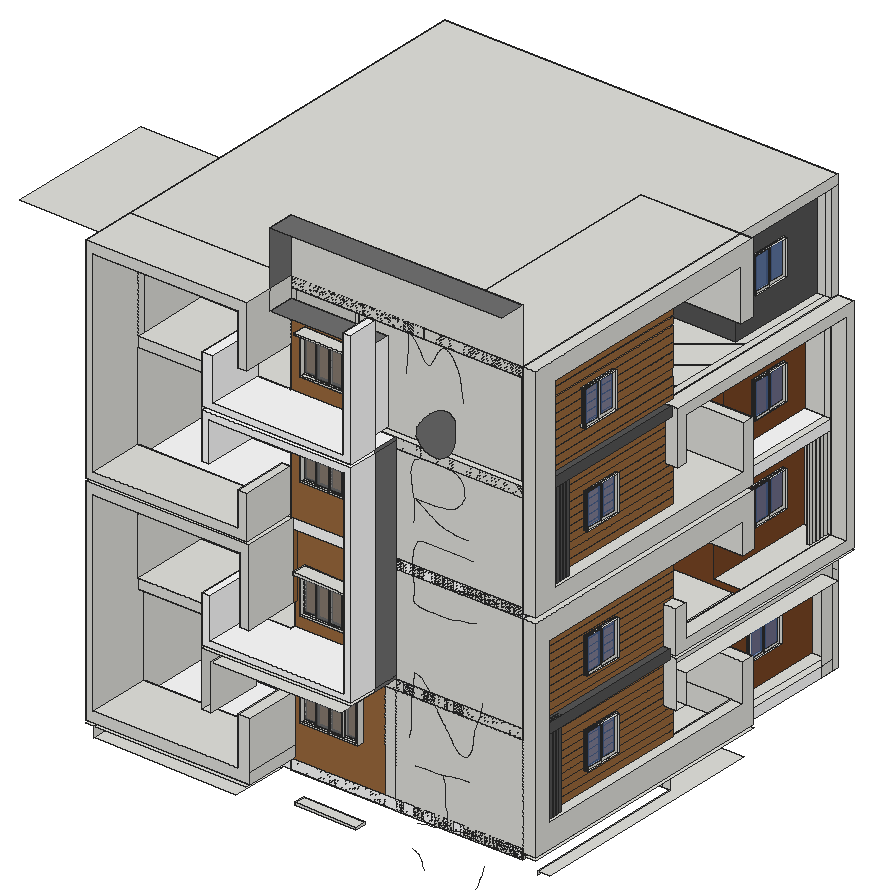
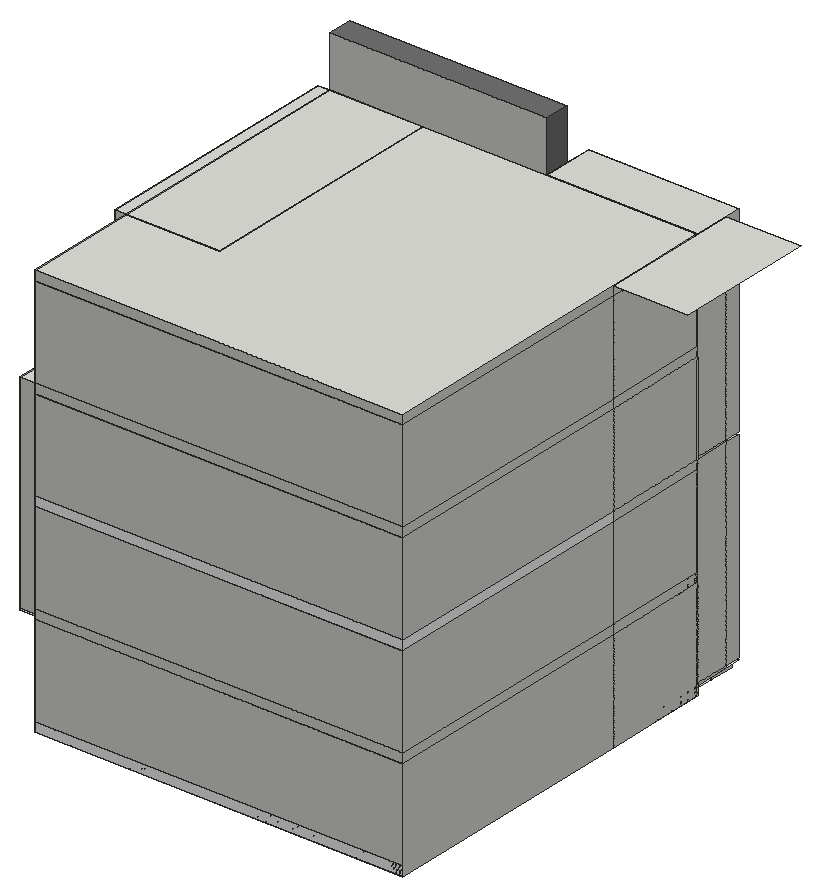
# SketchUp Ruby script. Lengths in inches.
U = 1.inch
M = Sketchup.active_model
def pt(a) = Geom::Point3d.new(a.map { |v| v * U })
def face(e, loops, mat)
  f = e.add_face(loops[0].map { |a| pt(a) })
  loops[1..].each { |l| e.add_face(l.map { |a| pt(a) }).erase! }
  f.material = f.back_material = mat if mat
  f
end
# faces: each face lists its corners as indices into pts; further lists are holes
def faces(e, pts, list, mat = nil) = list.each { |f| face(e, (f[0].is_a?(Array) ? f : [f]).map { |l| l.map { |i| pts[i] } }, mat) }
# xy, xz, yz: faces in a plane at the given z, y or x. An outline is a flat list of corners, or four numbers for a rectangle; further outlines are holes
def ring(l) = l.size == 4 ? [[l[0], l[1]], [l[2], l[1]], [l[2], l[3]], [l[0], l[3]]] : l.each_slice(2).to_a
def flat(e, list, mat, &to3) = list.each { |f| face(e, (f[0].is_a?(Array) ? f : [f]).map { |l| ring(l).map { |u, v| to3.(u, v) } }, mat) }
def xy(e, z, list, mat = nil) = flat(e, list, mat) { |x, y| [x, y, z] }
def xz(e, y, list, mat = nil) = flat(e, list, mat) { |x, z| [x, y, z] }
def yz(e, x, list, mat = nil) = flat(e, list, mat) { |y, z| [x, y, z] }
def lines(e, pts, list) = list.each { |a, b| e.add_line(pt(pts[a]), pt(pts[b])) }
# prism: a flat outline (further loops are holes) pulled along v
def prism(e, loops, v, mat = nil)
  f = face(e, loops, mat); d = Geom::Vector3d.new(v.map { |x| x * U })
  f.pushpull(f.normal.samedirection?(d) ? d.length : -d.length)
end
def box(e, o, s, mat = nil) = prism(e, [[o, [o[0] + s[0], o[1], o[2]], [o[0] + s[0], o[1] + s[1], o[2]], [o[0], o[1] + s[1], o[2]]]], [0, 0, s[2]], mat)
def at(x, y, z, deg = 0) = Geom::Transformation.translation(pt([x, y, z])) * Geom::Transformation.rotation(ORIGIN, Z_AXIS, deg.degrees)
def axes(o, x, y, z) = Geom::Transformation.new([*x, 0, *y, 0, *z, 0, *pt(o).to_a, 1])
def part(name) = M.definitions.add(name)
# library, detail: a bought-in or finely detailed component or shape, given as its bounding box
def library(name, o, s) = part(name).tap { |d| box(d.entities, o, s) }
def detail(e, o, s) = box(e.add_group.entities, o, s)
def put(e, d, t, mat = nil) = e.add_instance(d, t).tap { |i| i.material = mat if mat }
def group(e, t, mat = nil) = e.add_group.tap { |g| g.transformation = t; g.material = mat if mat }.entities
root = M.entities
M.materials.add("[Color M00]").color = [255, 255, 255]
M.materials.add("[Color M05]").color = [114, 114, 114]
M.materials.add("[Color M06]").color = [86, 86, 86]
M.materials.add("[Translucent Glass Blue]").color = [100, 149, 237]
M.materials["[Translucent Glass Blue]"].alpha = 0.5
M.materials.add("[Translucent_Glass_Gray]").color = [128, 128, 128]
M.materials["[Translucent_Glass_Gray]"].alpha = 0.5
M.materials.add("[Wood Floor]").color = [155, 105, 61]
M.materials.add("[Wood Veneer 01]").color = [120, 70, 37]
M.materials.add("[Wood Veneer 02]").color = [190, 128, 91]
c1 = part("Group\#4")
box(c1.entities,[0,-480,0],[480,480,12])
c2 = part("Janela aluminio")
xy(c2.entities,0,[[0,0,47.24,1.57],[23.62,1.57,47.24,2.76],[0,2.76,25.98,3.9375],[0,3.9375,47.24,5.91]])
xy(c2.entities,43.31,[[0,0,47.24,1.57],[23.62,1.57,47.24,2.76],[0,2.76,0,5.91,47.24,5.91,47.24,3.9375,25.98,3.9375,25.98,2.76],[25.98,2.76,47.24,3.9375]])
xz(c2.entities,1.57,[[0,0,23.62,0,23.62,41.34,21.26,41.34,21.26,1.97,1.97,1.97,1.97,41.34,23.62,41.34,23.62,43.31,0,43.31],[[23.62,0,47.24,43.31],[25.7,1.97,45.28,41.34]]])
xz(c2.entities,2.76,[[[0,0,23.62,43.31],[2.36,2.36,21.26,40.94]],[23.62,0,25.98,43.31]])
xz(c2.entities,2.76,[[2.36,2.36,21.26,40.94]],"[Translucent Glass Blue]")
xz(c2.entities,3.9375,[[25.98,0,25.98,2.36,44.88,2.36,44.88,40.94,25.98,40.94,25.98,43.31,47.24,43.31,47.24,0]])
xz(c2.entities,3.9375,[[25.98,2.36,44.88,40.94]],"[Translucent Glass Blue]")
yz(c2.entities,0,[[0,0,1.57,43.31],[2.76,0,5.91,43.31]])
yz(c2.entities,23.62,[[1.57,0,2.76,43.31]])
yz(c2.entities,25.98,[[2.76,0,3.9375,43.31]])
yz(c2.entities,47.24,[[0,0,1.57,43.31],[1.57,0,2.76,43.31],[3.9375,0,5.91,43.31]])
c3 = part("Group\#11")
box(c3.entities,[0,0,0],[3.1875,2.5625,106.5625],"[Color M06]")
c4 = part("Group\#5")
xy(c4.entities,0,[[0,0,3.25,201.7]])
xy(c4.entities,8.11,[[0,0,3.25,201.7]])
xz(c4.entities,201.7,[[0,0,3.25,8.11]])
yz(c4.entities,3.25,[[0,0,201.7,8.11]])
c5 = part("Window frame")
prism(c5.entities,[[[0,70.87,0],[0,0,0],[0,0,47.24],[0,70.87,47.24]],[[0,1.97,1.97],[0,68.9,1.97],[0,68.9,45.28],[0,1.97,45.28]]],[7.875,0,0])
c6 = part("Window sash")
xy(c6.entities,0,[[0,0,3.9375,16.73]])
xy(c6.entities,0.98,[[0,0.98,1.77,15.75],[1.77,0.98,2.85,15.75],[2.85,0.98,3.9375,15.75]])
xy(c6.entities,42.32,[[0,0.98,1.77,15.75],[1.77,0.98,2.85,15.75],[2.85,0.98,3.9375,15.75]])
xy(c6.entities,43.31,[[0,0,3.9375,16.73]])
xz(c6.entities,0,[[0,0,3.9375,43.31]])
xz(c6.entities,0.98,[[0,0.98,1.77,42.32],[1.77,0.98,2.85,42.32],[2.85,0.98,3.9375,42.32]])
xz(c6.entities,15.75,[[0,0.98,1.77,42.32],[1.77,0.98,2.85,42.32],[2.85,0.98,3.9375,42.32]])
xz(c6.entities,16.73,[[0,0,3.9375,43.31]])
yz(c6.entities,0,[[[0,0,16.73,43.31],[0.98,0.98,15.75,42.32]]])
yz(c6.entities,1.77,[[0.98,0.98,15.75,42.32]],"[Translucent_Glass_Gray]")
yz(c6.entities,2.85,[[0.98,0.98,15.75,42.32]],"[Translucent_Glass_Gray]")
yz(c6.entities,3.9375,[[[0,0,16.73,43.31],[0.98,0.98,15.75,42.32]]])
c7 = part("simple window")
p = [[0,68.9,1.97],[0,35.43,1.97]]
lines(c7.entities,p,[[0,1]])
put(c7.entities,c5,at(0,0,0))
put(c7.entities,c6,axes([1.14,52.17,1.97],[0.71,0,0],[0,1,0],[0,0,1]))
put(c7.entities,c6,axes([1.14,1.97,1.97],[0.71,0,0],[0,1,0],[0,0,1]))
put(c7.entities,c6,axes([3.9375,18.7,1.97],[0.71,0,0],[0,1,0],[0,0,1]))
put(c7.entities,c6,axes([3.9375,35.43,1.97],[0.71,0,0],[0,1,0],[0,0,1]))
c8 = part("Group\#12")
box(c8.entities,[0,0,-113.625],[4.125,3.0625,113.625])
prism(root,[[[309.42,176.67,224.48],[385.14,174.47,224.48],[384.74,160.72,224.48],[309.02,162.93,224.48]]],[0,0,2.95])
prism(root,[[[310.01,176.625,477.8],[385.52,174.46,477.8],[385.01,156.71,477.8],[309.5,158.88,477.8]]],[0,0,3.17])
prism(root,[[[309.78,176.625,739.55],[382.52,174.54,739.55],[382.09,159.42,739.55],[309.34,161.5,739.55]]],[0,0,2.58])
xy(root,230.57,[[576.8125,198.69,576.8125,400.39,441.125,400.39,441.125,495.37,591.75,495.37,591.75,198.69]])
xy(root,251.42,[[282.85,105.86,106.76,108.5,107.25,141,107.25,141.5625,107.78,176.625,283.87,173.99],[106.75,108.5,107.25,141.5625,107.25,141,106.76,108.5]])
xy(root,252,[[96.8125,176.625,96.8125,656.625,576.8125,656.625,576.8125,647.625,441.125,647.625,441.125,400.39,576.8125,400.39,576.8125,176.625,293.58,176.625,293.58,273.5625,105.8125,273.5625,105.8125,176.625],[441.125,400.39,576.8125,509.52],[441.125,509.52,552.625,647.625]])
xy(root,256.375,[[576.8125,176.625,591.75,509.52]])
xy(root,260.25,[[576.8125,176.625,591.75,508.3125]])
xy(root,264,[[294.92,105.68,295.94,173.81,107.78,176.625,107.25,176.625,107.25,108.5,106.76,108.5],[96.8125,108.5,106.75,108.5,107.25,141.5625,107.25,176.625,96.8125,176.625],[106.75,108.5,106.76,108.5,107.25,141,107.25,141.5625],[106.76,108.5,107.25,108.5,107.25,141],[105.8125,176.625,107.25,176.75],
  [368.4,185.625,567.8125,185.625,567.8125,391.39,432.125,391.39,432.125,647.625,105.8125,647.625,105.8125,282.5625,368.4,282.5625],[441.125,400.39,567.8125,493.4],[567.8125,400.39,576.8125,493.4],[441.125,493.4,567.8125,508.3125],[567.8125,493.4,576.8125,508.3125],
  [441.125,508.3125,552.625,647.625],[552.625,508.3125,567.8125,647.625],[567.8125,508.3125,576.8125,647.625]])
xy(root,266.9,[[96.8125,108.5,297.75,176.625],[105.8125,176.625,297.75,185.625]])
xy(root,280.02,[[105.8125,108.5,282.85,185.625]])
xy(root,289.03,[[576.8125,196.5,591.75,493.4]])
xy(root,328.5625,[[238.96,108.5,250.4375,176.625]])
xy(root,331.1,[[576.8125,385.5625,596.375,400.39]])
xy(root,335.41,[[441.125,493.4,591.75,508.3125]])
xy(root,338.39,[[282.85,108.5,297.75,185.625]])
xy(root,365.16,[[576.8125,400.39,596.375,631.75]])
xy(root,384,[[250.4375,108.5,408.47,176.625],[[96.8125,176.625,105.8125,176.625,105.8125,273.5625,293.58,273.5625,293.58,176.625,576.8125,176.625,576.8125,400.39,441.125,400.39,441.125,508.3125,552.625,508.3125,552.625,647.625,576.8125,647.625,576.8125,656.625,96.8125,656.625],[368.4,185.625,368.4,282.5625,105.8125,282.5625,105.8125,647.625,432.125,647.625,432.125,391.39,567.8125,391.39,567.8125,185.625]]])
xy(root,384,[[576.8125,196.5,589.1875,385.5625]],"[Color M06]")
xy(root,387.92,[[576.8125,385.5625,596.375,656.625]])
xy(root,390.25,[[576.8125,385.5625,596.375,656.7]])
xy(root,396,[[238.96,108.5,421.4,176.625],[[96.8125,176.625,105.8125,176.625,105.8125,273.5625,293.58,273.5625,293.58,176.625,576.8125,176.625,576.8125,400.39,441.125,400.39,441.125,508.3125,576.8125,508.3125,576.8125,656.625,96.8125,656.625],[368.4,185.625,368.4,282.5625,105.8125,282.5625,105.8125,647.625,432.125,647.625,432.125,391.39,567.8125,391.39,567.8125,185.625]],[105.8125,176.625,293.58,273.5625],[368.4,185.625,567.8125,185.625,567.8125,391.39,432.125,391.39,432.125,647.625,105.8125,647.625,105.8125,282.5625,368.4,282.5625],[441.125,400.39,567.8125,508.3125],
  [567.8125,400.39,576.8125,508.3125]])
xy(root,396,[[576.8125,196.5,589.1875,385.5625]],"[Color M06]")
xy(root,399.23,[[238.96,108.5,421.4,176.625]],"[Color M00]")
xy(root,402.375,[[576.8125,400.39,596.375,645.5],[543.8125,508.3125,576.8125,645.5]])
xy(root,406.73,[[248.78,108.5,412.35,108.5,412.35,181.6875,293.58,181.6875,293.58,176.625,248.78,176.625]],"[Color M00]")
xy(root,434.5625,[[284.9,108.5,295.8125,176.625]])
xy(root,434.5625,[[293.58,176.625,295.8125,181.6875]],"[Wood Floor]")
xy(root,442.24,[[576.8125,385.5625,596.375,400.39]])
xy(root,451.24,[[443.1875,493.73,591.75,509.52]])
xy(root,455.73,[[238.96,108.5,248.78,176.625]],"[Color M00]")
xy(root,488.49,[[576.8125,196.5,576.8125,400.39,443.1875,400.39,443.1875,493.73,591.75,493.73,591.75,196.5]])
xy(root,516,[[105.8125,108.5,284.9,176.625],[[96.8125,176.625,105.8125,176.625,105.8125,273.5625,293.58,273.5625,293.58,176.625,295.8125,176.625,295.8125,181.6875,412.35,181.6875,412.35,176.625,576.8125,176.625,576.8125,400.39,441.125,400.39,441.125,508.3125,543.8125,508.3125,543.8125,645.5,576.8125,645.5,576.8125,656.625,96.8125,656.625],[368.4,185.625,368.4,282.5625,105.8125,282.5625,105.8125,647.625,432.125,647.625,432.125,391.39,567.8125,391.39,567.8125,185.625]],[105.8125,176.625,293.58,273.5625]])
xy(root,516.375,[[576.8125,176.625,591.75,176.625,591.75,509.52,443.1875,509.52,443.1875,400.39,576.8125,400.39]])
xy(root,522,[[576.8125,176.625,591.75,508.3125]])
xy(root,528,[[96.8125,108.5,295.8125,176.625],[[96.8125,176.625,105.8125,176.625,105.8125,273.5625,293.58,273.5625,293.58,176.625,576.8125,176.625,576.8125,400.39,441.125,400.39,441.125,524.01,543.8125,524.01,543.8125,647.625,576.8125,647.625,576.8125,656.625,96.8125,656.625],[368.4,185.625,368.4,282.5625,105.8125,282.5625,105.8125,647.625,432.125,647.625,432.125,391.39,567.8125,391.39,567.8125,185.625]],[368.4,185.625,567.8125,185.625,567.8125,391.39,432.125,391.39,432.125,647.625,105.8125,647.625,105.8125,282.5625,368.4,282.5625],[441.125,400.39,452.75,400.39,452.75,508.3125,567.8125,508.3125,567.8125,647.625,543.8125,647.625,543.8125,524.01,441.125,524.01],[452.75,400.39,567.8125,508.3125],
  [567.8125,400.39,576.8125,508.3125],[567.8125,508.3125,576.8125,647.625]])
xy(root,531.25,[[96.8125,108.5,293.58,176.625]])
xy(root,541.94,[[105.8125,108.5,282.6,176.625]])
xy(root,542.625,[[576.8125,206.2,591.75,206.2,591.75,494.4,452.75,494.4,452.75,400.39,576.8125,400.39]])
xy(root,583.51,[[282.6,108.5,293.58,176.625]])
xy(root,595.125,[[576.8125,388.1875,596.375,400.39]])
xy(root,596.1875,[[452.75,494.4,591.75,508.3125]])
xy(root,599.8125,[[238.96,108.5,247.93,176.625]],"[Color M00]")
xy(root,648,[[[96.8125,176.625,105.8125,176.625,105.8125,273.5625,293.58,273.5625,293.58,176.625,576.8125,176.625,576.8125,400.39,441.125,400.39,441.125,524.01,543.8125,524.01,543.8125,647.625,576.8125,647.625,576.8125,656.625,96.8125,656.625],[368.4,185.625,368.4,282.5625,105.8125,282.5625,105.8125,647.625,432.125,647.625,432.125,391.39,567.8125,391.39,567.8125,185.625]],[576.8125,400.39,596.375,645.5]])
xy(root,648,[[247.93,108.5,412.35,176.625]],"[Color M00]")
xy(root,648,[[576.8125,206.2,588.625,388.1875]],"[Color M06]")
xy(root,656.3125,[[238.96,108.5,421.4,176.625]],"[Color M00]")
xy(root,660,[[[96.8125,176.625,105.8125,176.625,105.8125,273.5625,293.58,273.5625,293.58,176.625,576.8125,176.625,576.8125,400.39,441.125,400.39,441.125,524.01,558.6875,524.01,558.6875,647.625,576.8125,647.625,576.8125,656.625,96.8125,656.625],[368.4,185.625,368.4,282.5625,105.8125,282.5625,105.8125,647.625,432.125,647.625,432.125,391.39,567.8125,391.39,567.8125,185.625]],[105.8125,176.625,293.58,273.5625],[368.4,185.625,567.8125,185.625,567.8125,391.39,432.125,391.39,432.125,647.625,105.8125,647.625,105.8125,282.5625,368.4,282.5625],[576.8125,388.1875,596.375,656.7],[441.125,400.39,567.8125,400.39,567.8125,647.625,558.6875,647.625,558.6875,524.01,441.125,524.01],
  [567.8125,400.39,576.8125,647.625]])
xy(root,660,[[576.8125,206.2,588.625,388.1875]],"[Color M06]")
xy(root,660.31,[[238.96,108.5,421.4,176.625]],"[Color M00]")
xy(root,667.83,[[252.22,108.5,411.47,176.625]],"[Color M00]")
xy(root,706.5625,[[455.0625,490.39,591.75,508.3125]])
xy(root,717.3125,[[283.44,108.5,293.58,176.625]])
xy(root,719.51,[[238.96,108.5,252.22,176.625]],"[Color M00]")
xy(root,767.74,[[293.58,144.25,411.47,176.625]],"[Color M05]")
xy(root,768.8125,[[576.8125,206.2,576.8125,400.39,455.0625,400.39,455.0625,490.39,591.75,490.39,591.75,206.2]])
xy(root,780,[[105.8125,108.5,283.44,176.625],[96.8125,176.625,105.8125,176.625,105.8125,273.5625,293.58,273.5625,293.58,176.625,455.0625,176.625,455.0625,185.625,368.4,185.625,368.4,282.5625,105.8125,282.5625,105.8125,647.625,432.125,647.625,432.125,391.39,455.0625,391.39,455.0625,400.39,441.125,400.39,441.125,524.01,558.6875,524.01,558.6875,647.625,576.8125,647.625,576.8125,656.625,96.8125,656.625],[455.0625,176.625,576.8125,176.625,576.8125,400.39,455.0625,400.39,455.0625,391.39,567.8125,391.39,567.8125,185.625,455.0625,185.625],[455.0625,185.625,567.8125,391.39]])
xy(root,792,[[96.8125,108.5,293.58,176.625],[0,129.5,96.8125,313.4],[455.0625,176.625,591.75,508.3125]])
xy(root,801.24,[[411.47,108.5,421.4,144.25]],"[Color M00]")
xy(root,859.0625,[[293.58,144.25,576.8125,176.625]],"[Color M05]")
xz(root,108.5,[[96.8125,266.9,297.75,266.9,297.75,338.39,282.85,338.39,282.85,280.02,105.8125,280.02,105.8125,516,284.9,516,284.9,434.5625,295.8125,434.5625,295.8125,528,96.8125,528],[96.8125,531.25,293.58,531.25,293.58,583.51,282.6,583.51,282.6,541.94,105.8125,541.94,105.8125,780,283.44,780,283.44,717.3125,293.58,717.3125,293.58,792,96.8125,792]])
xz(root,108.5,[[238.96,399.23,421.4,399.23,421.4,656.3125,238.96,656.3125,238.96,599.8125,247.93,599.8125,247.93,648,412.35,648,412.35,406.73,248.78,406.73,248.78,455.73,238.96,455.73],[238.96,660.31,421.4,660.31,421.4,801.24,411.47,801.24,411.47,667.83,252.22,667.83,252.22,719.51,238.96,719.51]],"[Color M00]")
xz(root,144.25,[[499.28,678.61,502.39,679.59,504.6,680.79,507.3125,682.48,509.4,683.71,511.65,685.61,512.91,687.64,514.6,689.38,515.95,691.83,517.19,693.71,518.06,696.2,518.48,698.83,518.75,701.49,518.93,703.9,519.01,706.6,519.06,709.68,519.08,712.16,519.08,715.27,519.07,717.8,519.05,720.89,519.03,723.43,518.67,726.53,517.58,728.38,515.96,730.33,513.8,731.55,511.41,732.18,508.87,732.625,506.22,732.9,498.73,730.52,494.25,727.71,489.21,724.33,488.32,722.59,486.18,720.94,484.83,719.08,482.91,717.36,481.51,715.31,479.9,713.53,478.57,711.1,477,709.55,475.72,707.47,474.84,705.29,473.375,703.48,472.87,700.99,472.54,698.74,472.29,696.5,472.16,693.875,473.78,691.2,475.09,689.5,476.52,686.92,478.12,684.95,480.42,683.44,481.86,681.66,483.9,680.62,486.04,679.74,488.85,679.28,491.18,678.99,493.5,678.8,496.52,678.68]],"[Color M05]")
xz(root,176.625,[[96.8125,252,105.8125,264],[408.47,252,421.4,384],[421.4,252,576.8125,384],[576.8125,260.25,591.75,516.375],[96.8125,264,105.8125,266.9],
  [238.96,328.5625,238.96,396,421.4,396,421.4,384,250.4375,384,250.4375,328.5625],[96.8125,384,105.8125,396],[421.4,384,576.8125,396],[421.4,396,576.8125,516],[284.9,434.5625,293.58,516],
  [293.58,434.5625,295.8125,516],[96.8125,516,295.8125,528],[421.4,516,576.8125,528],[576.8125,522,591.75,792],[96.8125,528,105.8125,531.25],
  [421.4,528,576.8125,648],[105.8125,531.25,105.8125,541.94,282.6,541.94,282.6,583.51,293.58,583.51,293.58,531.25],[96.8125,648,105.8125,660],[421.4,648,576.8125,660],[96.8125,660,105.8125,780],
  [283.44,717.3125,283.44,780,96.8125,780,96.8125,792,293.58,792,293.58,717.3125],[293.58,780,293.58,859.0625,576.8125,859.0625,576.8125,792,455.0625,792,455.0625,780],[455.0625,780,576.8125,792]])
xz(root,176.625,[[412.35,516,421.4,528],[238.96,599.8125,238.96,656.3125,421.4,656.3125,421.4,648,247.93,648,247.93,599.8125]],"[Color M00]")
xz(root,176.625,[[293.58,252,408.47,384],[293.58,396,421.4,399.23],[238.96,399.23,238.96,455.73,248.78,455.73,248.78,406.73,293.58,406.73,293.58,399.23],[293.58,528,412.35,648],[412.35,528,421.4,648],
  [293.58,660,421.4,660.31],[238.96,660.31,238.96,719.51,252.22,719.51,252.22,667.83,293.58,667.83,293.58,660.31],[293.58,667.83,411.47,767.74]],"[Wood Floor]")
xz(root,181.6875,[[293.58,406.73,412.35,406.73,412.35,516,295.8125,516,295.8125,434.5625,293.58,434.5625]],"[Wood Floor]")
xz(root,185.625,[[368.4,252,567.8125,264],[368.4,264,567.8125,384],[105.8125,266.9,105.8125,280.02,282.85,280.02,282.85,338.39,293.58,338.39,293.58,266.9],[293.58,266.9,297.75,280.02],[293.58,280.02,297.75,338.39],
  [368.4,396,567.8125,516],[368.4,528,567.8125,648],[368.4,660,567.8125,780]])
xz(root,196.5,[[576.8125,289.03,576.8125,384,589.1875,384,589.1875,396,576.8125,396,576.8125,488.49,591.75,488.49,591.75,289.03],[576.8125,384,589.1875,396]])
xz(root,206.2,[[576.8125,542.625,576.8125,648,588.625,648,588.625,660,576.8125,660,576.8125,768.8125,591.75,768.8125,591.75,542.625],[576.8125,648,588.625,660]])
xz(root,273.5625,[[105.8125,252,293.58,384],[105.8125,396,293.58,516],[105.8125,528,293.58,648],[105.8125,660,293.58,780]])
xz(root,282.5625,[[105.8125,252,368.4,264],[105.8125,264,368.4,384],[105.8125,396,368.4,516],[105.8125,528,368.4,648],[105.8125,660,368.4,780]])
xz(root,385.5625,[[576.8125,331.1,596.375,331.1,596.375,387.92,589.1875,387.92,589.1875,384,576.8125,384],[576.8125,384,589.1875,387.92],[576.8125,387.92,589.1875,390.25],[576.8125,390.25,589.1875,396],[589.1875,390.25,596.375,390.25,596.375,442.24,576.8125,442.24,576.8125,396,589.1875,396]])
xz(root,388.1875,[[576.8125,595.125,596.375,595.125,596.375,660,588.625,660,588.625,648,576.8125,648],[576.8125,648,588.625,660]])
xz(root,391.39,[[432.125,252,562.8125,264],[562.8125,252,567.8125,264],[432.125,264,562.8125,384],[562.8125,264,567.8125,384],[432.125,396,562.8125,516],
  [562.8125,396,567.8125,516],[432.125,528,562.8125,648],[562.8125,528,567.8125,648],[432.125,660,562.8125,780],[562.8125,660,567.8125,780]])
xz(root,400.39,[[441.125,230.57,567.8125,252],[567.8125,230.57,576.8125,252],[441.125,252,567.8125,264],[567.8125,252,576.8125,264],[441.125,264,567.8125,384],
  [567.8125,264,576.8125,384],[576.8125,331.1,596.375,365.16],[441.125,396,441.125,516,443.1875,516,443.1875,488.49,567.8125,488.49,567.8125,396],[567.8125,396,576.8125,488.49],[576.8125,402.375,596.375,442.24],
  [443.1875,488.49,567.8125,516],[567.8125,488.49,576.8125,516],[443.1875,516,576.8125,516.375],[441.125,528,441.125,648,567.8125,648,567.8125,542.625,452.75,542.625,452.75,528],[452.75,528,567.8125,542.625],
  [567.8125,528,576.8125,542.625],[567.8125,542.625,576.8125,648],[576.8125,595.125,596.375,648],[441.125,660,441.125,780,455.0625,780,455.0625,768.8125,567.8125,768.8125,567.8125,660],[567.8125,660,576.8125,768.8125],
  [455.0625,768.8125,567.8125,780],[567.8125,768.8125,576.8125,780]])
xz(root,490.39,[[455.0625,706.5625,591.75,768.8125]])
xz(root,493.4,[[441.125,264,576.8125,289.03],[441.125,289.03,591.75,335.41]])
xz(root,493.73,[[443.1875,451.24,591.75,488.49]])
xz(root,494.4,[[452.75,542.625,591.75,596.1875]])
xz(root,508.3125,[[576.8125,260.25,576.8125,264,552.625,264,552.625,335.41,591.75,335.41,591.75,260.25],[441.125,264,552.625,335.41],[576.8125,522,576.8125,528,452.75,528,452.75,596.1875,591.75,596.1875,591.75,522],[455.0625,706.5625,591.75,792]])
xz(root,508.3125,[[441.125,335.41,552.625,384],[441.125,396,576.8125,396,576.8125,402.375,543.8125,402.375,543.8125,516,441.125,516]],"[Wood Veneer 01]")
xz(root,509.52,[[443.1875,451.24,591.75,516.375]])
xz(root,524.01,[[441.125,660,558.6875,780]],"[Color M06]")
xz(root,524.01,[[441.125,528,543.8125,648]],"[Wood Veneer 01]")
xz(root,645.5,[[543.8125,402.375,576.8125,516],[576.8125,402.375,596.375,648]])
xz(root,647.625,[[105.8125,252,432.125,264],[441.125,252,567.8125,264],[567.8125,252,576.8125,264],[105.8125,264,432.125,384],[552.625,264,567.8125,384],
  [567.8125,264,576.8125,384],[105.8125,396,432.125,516],[105.8125,528,432.125,648],[543.8125,528,567.8125,648],[567.8125,528,576.8125,648],
  [105.8125,660,432.125,780],[558.6875,660,567.8125,780],[567.8125,660,576.8125,780]])
xz(root,656.625,[[96.8125,252,576.8125,384],[96.8125,396,576.8125,516],[96.8125,528,576.8125,648],[96.8125,660,576.8125,780]])
xz(root,656.7,[[576.8125,390.25,596.375,660]])
yz(root,96.8125,[[176.625,252,176.75,384],[176.75,252,313.4,384],[313.4,252,656.625,384],[129.5,264,176.625,266.9],[108.5,266.9,129.5,528],
  [129.5,266.9,176.625,528],[176.625,384,176.75,396],[176.75,384,313.4,396],[176.625,396,176.75,516],[176.75,396,313.4,516],
  [313.4,396,656.625,516],[176.625,516,176.75,528],[176.75,516,313.4,528],[129.5,528,176.625,531.25],[176.625,528,176.75,648],
  [176.75,528,313.4,648],[313.4,528,656.625,648],[108.5,531.25,129.5,792],[129.5,531.25,176.625,792],[176.625,648,176.75,660],
  [176.75,648,313.4,660],[176.625,660,176.75,780],[176.75,660,313.4,780],[313.4,660,656.625,780],[176.625,780,176.75,792],
  [176.75,780,313.4,792]])
yz(root,105.8125,[[176.625,252,176.75,264],[176.75,252,185.625,252,185.625,266.9,176.625,266.9,176.625,264,176.75,264],[185.625,252,273.5625,384],[282.5625,252,647.625,264],[282.5625,264,647.625,384],
  [108.5,280.02,185.625,280.02,185.625,384,176.625,384,176.625,516,108.5,516],[176.625,396,273.5625,516],[282.5625,396,647.625,516],[176.625,528,273.5625,648],[282.5625,528,647.625,648],
  [108.5,541.94,176.625,780],[176.625,660,185.625,780],[185.625,660,273.5625,780],[282.5625,660,647.625,780]])
yz(root,107.25,[[108.5,251.42,141.5625,264]])
yz(root,238.96,[[108.5,328.5625,176.625,396]])
yz(root,238.96,[[108.5,399.23,176.625,455.73],[108.5,599.8125,176.625,656.3125],[108.5,660.31,176.625,719.51]],"[Color M00]")
yz(root,247.93,[[108.5,599.8125,176.625,648]],"[Color M00]")
yz(root,248.78,[[108.5,406.73,176.625,455.73]],"[Color M00]")
yz(root,250.4375,[[108.5,328.5625,176.625,384]])
yz(root,252.22,[[108.5,667.83,176.625,719.51]],"[Color M00]")
yz(root,282.6,[[108.5,541.94,176.625,583.51]])
yz(root,282.85,[[108.5,280.02,185.625,338.39]])
yz(root,283.44,[[108.5,717.3125,176.625,780]])
yz(root,284.9,[[108.5,434.5625,176.625,516]])
yz(root,293.58,[[176.625,252,185.625,384],[185.625,252,273.5625,384],[176.625,396,176.625,406.73,181.6875,406.73,181.6875,434.5625,176.625,434.5625,176.625,516,185.625,516,185.625,396],[185.625,396,273.5625,516],[176.625,528,185.625,648],
  [185.625,528,273.5625,648],[108.5,531.25,176.625,583.51],[176.625,660,185.625,780],[185.625,660,273.5625,780],[108.5,717.3125,176.625,717.3125,176.625,767.74,144.25,767.74,144.25,792,108.5,792],
  [144.25,767.74,176.625,792]])
yz(root,293.58,[[144.25,792,176.625,859.0625]],"[Color M05]")
yz(root,295.8125,[[108.5,434.5625,176.625,528]])
yz(root,295.8125,[[176.625,434.5625,181.6875,516]],"[Wood Floor]")
yz(root,297.75,[[108.5,266.9,185.625,280.02],[108.5,280.02,185.625,338.39]])
yz(root,368.4,[[185.625,252,282.5625,264],[185.625,264,282.5625,384],[185.625,396,282.5625,516],[185.625,528,282.5625,648],[185.625,660,282.5625,780]])
yz(root,411.47,[[108.5,667.83,108.5,801.24,144.25,801.24,144.25,767.74,176.625,767.74,176.625,667.83]],"[Color M00]")
yz(root,412.35,[[108.5,406.73,108.5,648,176.625,648,176.625,516,181.6875,516,181.6875,406.73]],"[Color M00]")
yz(root,421.4,[[108.5,399.23,144.25,656.3125],[108.5,660.31,144.25,801.24]],"[Color M00]")
yz(root,421.4,[[144.25,396,176.625,399.23],[144.25,399.23,176.625,656.3125],[144.25,656.3125,176.625,660.31]],"[Color M05]")
yz(root,432.125,[[391.39,252,647.625,264],[391.39,264,647.625,384],[391.39,396,647.625,516],[391.39,528,647.625,648],[391.39,660,647.625,780]])
yz(root,441.125,[[400.39,252,647.625,264]])
yz(root,441.125,[[400.39,264,493.4,264,493.4,335.41,508.3125,335.41,508.3125,384,400.39,384],[400.39,396,508.3125,516],[400.39,528,524.01,648],[400.39,660,524.01,780]],"[Wood Veneer 02]")
yz(root,443.1875,[[493.73,451.24,493.73,488.49,400.39,488.49,400.39,516.375,509.52,516.375,509.52,451.24]])
yz(root,452.75,[[400.39,528,400.39,542.625,494.4,542.625,494.4,596.1875,508.3125,596.1875,508.3125,528]])
yz(root,455.0625,[[490.39,706.5625,490.39,768.8125,400.39,768.8125,400.39,780,176.625,780,176.625,792,508.3125,792,508.3125,706.5625]])
yz(root,543.8125,[[508.3125,402.375,645.5,516],[524.01,528,647.625,648]],"[Wood Veneer 01]")
yz(root,552.625,[[508.3125,264,647.625,384]],"[Wood Veneer 01]")
yz(root,558.6875,[[524.01,660,647.625,780]],"[Color M06]")
yz(root,567.8125,[[185.625,252,391.39,264],[185.625,264,391.39,384],[185.625,396,391.39,516],[185.625,528,391.39,648],[185.625,660,391.39,780]])
yz(root,576.8125,[[198.69,226.34,400.39,230.57],[176.625,252,400.39,256.375],[400.39,252,509.52,256.375],[631.75,252,647.625,264],[647.625,252,656.625,384],
  [176.625,256.375,400.39,260.25],[400.39,260.25,508.3125,264],[400.39,264,493.4,289.03],[631.75,264,631.75,365.16,400.39,365.16,400.39,384,647.625,384,647.625,264],[196.5,289.03,400.39,289.03,400.39,331.1,385.5625,331.1,385.5625,384,196.5,384],
  [385.5625,331.1,400.39,384],[176.625,384,196.5,396],[385.5625,384,656.625,387.92],[385.5625,390.25,385.5625,396,656.625,396,656.625,660,656.7,660,656.7,390.25],[176.625,396,196.5,396,196.5,488.49,400.39,488.49,400.39,516,176.625,516],
  [196.5,396,385.5625,396,385.5625,442.24,400.39,442.24,400.39,488.49,196.5,488.49],[385.5625,396,400.39,442.24],[400.39,396,508.3125,402.375],[508.3125,396,647.625,396,647.625,516,645.5,516,645.5,402.375,508.3125,402.375],[647.625,396,656.625,516],
  [176.625,516,400.39,516.375],[645.5,516,647.625,528],[647.625,516,656.625,528],[176.625,522,508.3125,528],[176.625,528,187.7,528,187.7,542.625,206.2,542.625,206.2,648,176.625,648],
  [187.7,528,400.39,542.625],[645.5,528,645.5,648,388.1875,648,388.1875,660,647.625,660,647.625,528],[647.625,528,656.625,648],[206.2,542.625,400.39,542.625,400.39,595.125,388.1875,595.125,388.1875,648,206.2,648],[388.1875,595.125,400.39,648],
  [176.625,648,206.2,660],[647.625,648,656.625,660],[176.625,660,206.2,660,206.2,768.8125,400.39,768.8125,400.39,780,176.625,780],[206.2,660,400.39,768.8125],[647.625,660,656.625,780]])
yz(root,588.625,[[206.2,648,388.1875,660]],"[Color M06]")
yz(root,589.1875,[[196.5,384,385.5625,396]],"[Color M06]")
yz(root,591.75,[[176.625,260.25,508.3125,260.25,508.3125,335.41,493.4,335.41,493.4,289.03,196.5,289.03,196.5,488.49,493.73,488.49,493.73,451.24,509.52,451.24,509.52,516.375,176.625,516.375],[176.625,522,508.3125,522,508.3125,596.1875,494.4,596.1875,494.4,542.625,206.2,542.625,206.2,768.8125,490.39,768.8125,490.39,706.5625,508.3125,706.5625,508.3125,792,176.625,792]])
yz(root,596.375,[[385.5625,390.25,656.7,390.25,656.7,660,388.1875,660,388.1875,595.125,400.39,595.125,400.39,648,645.5,648,645.5,402.375,400.39,402.375,400.39,442.24,385.5625,442.24]])
p = [[107.25,141.5625,264],[107.25,141.5625,251.42],[106.75,108.5,251.42],[106.75,108.5,264],[107.78,176.625,264],[293.58,176.625,264],
  [591.75,631.75,376.91],[595.1875,631.75,376.91],[460.4,144.25,757.46],[460.375,144.25,763.62],[460.91,144.25,769.2],[461.47,144.25,770.48],
  [461.62,144.25,773.59],[461.75,144.25,776.9],[461.85,144.25,779.34],[461.89,144.25,781.47],[461.91,144.25,784.14],[461.92,144.25,787.47],
  [461.93,144.25,789.61],[461.93,144.25,792.31],[461.92,144.25,795.06],[461.91,144.25,797.43],[461.91,144.25,799.78],[461.9,144.25,802.09],
  [462.56,144.25,804.6875],[465.38,144.25,802.68],[467.69,144.25,800.77],[469.18,144.25,799.12],[471.34,144.25,796.73],[472.49,144.25,794.56],
  [474.1,144.25,792.39],[475.43,144.25,790.5],[476.99,144.25,788.35],[478.27,144.25,786.51],[479.16,144.25,784.07],[480.3,144.25,781.51],
  [481.43,144.25,779.57],[483.2,144.25,778.01],[485.46,144.25,776.91],[488.23,144.25,776.01],[490.17,144.25,777.91],[491.38,144.25,780.43],
  [492.42,144.25,782.7],[493.94,144.25,784.6],[495.13,144.25,787.125],[495.95,144.25,789.38],[497.05,144.25,791.28],[498.125,144.25,793.8],
  [499.87,144.25,795.39],[500.76,144.25,797.48],[502.56,144.25,798.98],[504.51,144.25,800.64],[506.84,144.25,802],[509.37,144.25,800.93],
  [512,144.25,799.35],[514.03,144.25,797.0625],[515.97,144.25,796],[517.17,144.25,793.74],[518.83,144.25,791.28],[520.16,144.25,788.79],
  [521.0625,144.25,786.82],[522.56,144.25,784.92],[523.44,144.25,782.43],[524.2,144.25,779.87],[525.28,144.25,777.58],[526.01,144.25,774.94],
  [526.36,144.25,772.59],[526.625,144.25,769.95],[527.14,144.25,766.91],[527.32,144.25,764.46],[527.79,144.25,762.06],[527.97,144.25,759.35],
  [528.75,144.25,757.3125],[528.99,144.25,754.71],[529.49,144.25,752.375],[530.04,144.25,749.76],[468.98,144.25,598.37],[470.09,144.25,604.13],
  [470.07,144.25,609.89],[469.94,144.25,611.62],[470.02,144.25,613.8],[470.02,144.25,616.37],[470.01,144.25,618.65],[469.66,144.25,621.65],
  [469.24,144.25,624.46],[468.78,144.25,626.93],[467.92,144.25,630.0625],[467.31,144.25,632.59],[467.05,144.25,635.72],[466.84,144.25,638.63],
  [466.02,144.25,641.5],[465.81,144.25,644.39],[465.65,144.25,646.92],[465.51,144.25,650.05],[465.44,144.25,652.59],[466.07,144.25,654.69],
  [466.17,144.25,657.39],[467.25,144.25,660.1],[467.88,144.25,662.15],[468.79,144.25,664.81],[470.16,144.25,667.18],[472.28,144.25,668.47],
  [474.97,144.25,669.57],[477.21,144.25,670.49],[480.17,144.25,670.91],[483.29,144.25,671.2],[485.79,144.25,671.39],[488.6,144.25,671.5],
  [491.08,144.25,671.5625],[493.46,144.25,671.61],[496.16,144.25,671.63],[499.57,144.25,671.64],[502.11,144.25,671.65],[504.93,144.25,671.66],
  [507.78,144.25,671.66],[510.59,144.25,670.97],[513.76,144.25,670.84],[515.98,144.25,670.74],[518.73,144.25,669.61],[521.52,144.25,668.68],
  [523.27,144.25,667.34],[525.19,144.25,666.18],[526.73,144.25,664.36],[528.4375,144.25,662.03],[529.82,144.25,659.89],[530.44,144.25,657.34],
  [530.89,144.25,654.67],[531.2,144.25,651.95],[531.4,144.25,648.48],[531.52,144.25,646.22],[529.91,144.25,643.43],[528.95,144.25,641.27],
  [527.95,144.25,638.96],[526.48,144.25,636.97],[524.63,144.25,635.1],[522.67,144.25,632.92],[520.59,144.25,631.07],[518.09,144.25,629.6],
  [515.14,144.25,628.91],[512.74,144.25,627.41],[509.67,144.25,626.9],[506.82,144.25,626.58],[504,144.25,626.3125],[500.8,144.25,625.49],
  [497.89,144.25,625.27],[495.34,144.25,625.12],[492.86,144.25,624.99],[489.77,144.25,624.93],[486.95,144.25,624.89],[484.46,144.25,624.86],
  [481.67,144.25,624.85],[478.88,144.25,624.84],[476.09,144.25,624.84],[472.93,144.25,624.84],[470.375,144.25,624.84],[474.05,144.25,623.11],
  [475.92,144.25,621.39],[477.78,144.25,620.18],[480.42,144.25,618.55],[483.02,144.25,617.24],[485.37,144.25,615.3125],[488.08,144.25,612.9],
  [491.17,144.25,612.1],[494,144.25,610.12],[495.84,144.25,609.05],[498.17,144.25,607.52],[500.82,144.25,606.22],[503.8125,144.25,605.35],
  [506.28,144.25,604.19],[508.71,144.25,603.74],[511.45,144.25,603.45],[514.2,144.25,602.88],[516.98,144.25,602.35],[519.79,144.25,601.8],
  [522.28,144.25,601.58],[525.04,144.25,601.43],[527.83,144.25,601.32],[530.625,144.25,601.25],[533.79,144.25,601.21],[536.34,144.25,601.53],
  [541.33,144.25,580.27],[532.25,144.25,581.03],[524.7,144.25,581.03],[522.59,144.25,580.96],[519.6,144.25,581.02],[516.22,144.25,581.03],
  [513.22,144.25,581.03],[509.27,144.25,581.04],[505.12,144.25,581.04],[501.78,144.25,581.04],[498.04,144.25,581.04],[494.73,144.25,581.05],
  [490.64,144.25,581.05],[487.31,144.25,581.05],[483.18,144.25,581.05],[479.35,144.25,581.05],[476.03,144.25,580.15],[473.23,144.25,578.15],
  [471.96,144.25,574.94],[469.76,144.25,570.375],[468.92,144.25,567.58],[468.41,144.25,564.42],[468.02,144.25,561.24],[467.8125,144.25,558.18],
  [467.7,144.25,553.75],[467.625,144.25,550.42],[467.59,144.25,546.73],[467.58,144.25,542.93],[467.57,144.25,539.1875],[468.94,144.25,535.86],
  [469.23,144.25,532.16],[469.4375,144.25,527.51],[469.65,144.25,524.51],[469.76,144.25,520.33],[468.47,144.25,516.4375],[468.25,144.25,513.11],
  [470.375,144.25,510.26],[473.38,144.25,508.97],[476.45,144.25,508.09],[481.67,144.25,507.49],[485.15,144.25,507.16],[488.95,144.25,506.94],
  [492.4,144.25,507.26],[496.09,144.25,507.27],[501.2,144.25,507.27],[505.21,144.25,507.31],[508.72,144.25,507.3125],[511.7,144.25,507.32],
  [515.77,144.25,507.78],[519.06,144.25,507.87],[521.78,144.25,509.31],[524.87,144.25,510.11],[528.37,144.25,510.875],[531.92,144.25,511.25],
  [535.57,144.25,511.48],[539.28,144.25,512.1],[543,144.25,513.65],[545.85,144.25,514.05],[475.87,144.25,539.37],[488.74,144.25,539.36],
  [500.1,144.25,539.35],[501.08,144.25,539.35],[505.97,144.25,539.35],[509.55,144.25,539.34],[512.66,144.25,540.25],[516.4,144.25,540.89],
  [520.09,144.25,541.1],[523.33,144.25,541.3],[526.53,144.25,541.88],[530.14,144.25,542.04],[533.77,144.25,542.6],[537.45,144.25,542.78],
  [540.26,144.25,544.26],[463.23,144.25,361.1],[465.97,144.25,370.33],[465.94,144.25,378.64],[465.65,144.25,381.59],[465.86,144.25,385.04],
  [465.86,144.25,389.0625],[465.85,144.25,393.27],[465.86,144.25,397.07],[465.85,144.25,401.42],[465.83,144.25,405.85],[466.93,144.25,410.86],
  [467.6875,144.25,414.95],[468.49,144.25,418.36],[468.83,144.25,422.71],[469.04,144.25,426.54],[469.75,144.25,430.28],[469.93,144.25,434.05],
  [475.6,144.25,432.81],[479.04,144.25,431.11],[482.54,144.25,426.61],[485.26,144.25,423.76],[488.17,144.25,420.37],[489.94,144.25,416.74],
  [492.53,144.25,412.08],[495.19,144.25,406.03],[497.27,144.25,403.4375],[499.33,144.25,399.09],[502.44,144.25,395.14],[504.04,144.25,392],
  [507.1,144.25,388.875],[508.75,144.25,385.33],[511.77,144.25,382.33],[513.41,144.25,378.85],[516.4375,144.25,374.74],[517.52,144.25,371.05],
  [520.43,144.25,368.44],[523.09,144.25,365.48],[526.8,144.25,363.7],[530.86,144.25,362.79],[534.52,144.25,364.35],[537.66,144.25,368.82],
  [539.59,144.25,372.55],[540.64,144.25,376.11],[541.35,144.25,379.86],[541.77,144.25,383.55],[542.01,144.25,387.79],[543.26,144.25,392.7],
  [543.55,144.25,397.23],[545.4,144.25,401.26],[546.47,144.25,404.67],[547.4375,144.25,408.42],[549.5625,144.25,412.12],[550.73,144.25,416.33],
  [551.25,144.25,420.68],[552.22,144.25,424.54],[552.55,144.25,429.48],[470.73,144.25,332.42],[482.74,144.25,333.35],[491.0625,144.25,333.35],
  [495.41,144.25,333.25],[499.97,144.25,333.33],[504.37,144.25,333.89],[509.46,144.25,334.55],[513.59,144.25,335.86],[518.69,144.25,336.24],
  [523.41,144.25,337.07],[527.49,144.25,337.41],[532.62,144.25,337.59],[536.74,144.25,337.75],[507.75,144.25,324.08],[507.8,144.25,315.73],
  [507.84,144.25,306.46],[507.86,144.25,304.13],[507.88,144.25,300.23],[509.5625,144.25,296.62],[509.92,144.25,292.49],[510.17,144.25,288.68],
  [510.44,144.25,284.35],[510.58,144.25,279.34],[473.74,144.25,270.21],[483.93,144.25,273],[494.12,144.25,273],[496.62,144.25,273.83],
  [501.375,144.25,275.4],[505.82,144.25,275.79],[509.65,144.25,276.67],[514.68,144.25,277.04],[518.73,144.25,277.8],[523.2,144.25,278.63],
  [527.78,144.25,280.03],[531.21,144.25,281.02],[535.02,144.25,281.45],[538.8125,144.25,281.77],[543.07,144.25,281.98],[467.49,144.25,240.96],
  [474.93,144.25,237.25],[479.6,144.25,229.83],[479.61,144.25,226.12],[482.51,144.25,222.04],[544.86,144.25,223.6],[547.08,144.25,226.81],
  [548.39,144.25,231.54],[549.53,144.25,235.37],[551.77,144.25,239.71],[553.01,144.25,243.66],[554.13,144.25,248.04],[555.24,144.25,252.52]]
faces(root,p,[[0,1,2,3]])
lines(root,p,[[4,5],[6,7],[8,9],[9,10],[10,11],[11,12],[12,13],[13,14],[14,15],[15,16],[16,17],[17,18],
  [18,19],[19,20],[20,21],[21,22],[22,23],[23,24],[24,25],[25,26],[26,27],[27,28],[28,29],[29,30],
  [30,31],[31,32],[32,33],[33,34],[34,35],[35,36],[36,37],[37,38],[38,39],[39,40],[40,41],[41,42],
  [42,43],[43,44],[44,45],[45,46],[46,47],[47,48],[48,49],[49,50],[50,51],[51,52],[52,53],[53,54],
  [54,55],[55,56],[56,57],[57,58],[58,59],[59,60],[60,61],[61,62],[62,63],[63,64],[64,65],[65,66],
  [66,67],[67,68],[68,69],[69,70],[70,71],[71,72],[72,73],[73,74],[74,75],[76,77],[77,78],[78,79],
  [79,80],[80,81],[81,82],[82,83],[83,84],[84,85],[85,86],[86,87],[87,88],[88,89],[89,90],[90,91],
  [91,92],[92,93],[93,94],[94,95],[95,96],[96,97],[97,98],[98,99],[99,100],[100,101],[101,102],[102,103],
  [103,104],[104,105],[105,106],[106,107],[107,108],[108,109],[109,110],[110,111],[111,112],[112,113],[113,114],[114,115],
  [115,116],[116,117],[117,118],[118,119],[119,120],[120,121],[121,122],[122,123],[123,124],[124,125],[125,126],[126,127],
  [127,128],[128,129],[129,130],[130,131],[131,132],[132,133],[133,134],[134,135],[135,136],[136,137],[137,138],[138,139],
  [139,140],[140,141],[141,142],[142,143],[143,144],[144,145],[145,146],[146,147],[147,148],[148,149],[149,150],[150,151],
  [151,152],[152,153],[153,154],[154,155],[155,156],[156,157],[157,158],[158,159],[159,160],[160,161],[161,162],[162,163],
  [163,164],[164,165],[165,166],[166,167],[167,168],[168,169],[169,170],[170,171],[171,172],[172,173],[173,174],[174,175],
  [175,176],[176,177],[177,178],[178,179],[180,181],[181,182],[182,183],[183,184],[184,185],[185,186],[186,187],[187,188],
  [188,189],[189,190],[190,191],[191,192],[192,193],[193,194],[194,195],[195,196],[196,197],[197,198],[198,199],[199,200],
  [200,201],[201,202],[202,203],[203,204],[204,205],[205,206],[206,207],[207,208],[208,209],[209,210],[210,211],[211,212],
  [212,213],[213,214],[214,215],[215,216],[216,217],[217,218],[218,219],[219,220],[220,221],[221,222],[222,223],[223,224],
  [224,225],[225,226],[226,227],[227,228],[228,229],[229,230],[230,231],[231,232],[232,233],[233,234],[234,235],[235,236],
  [236,237],[208,238],[238,239],[239,240],[240,241],[241,242],[242,243],[243,244],[244,245],[245,246],[246,247],[247,248],
  [248,249],[249,250],[250,251],[251,252],[253,254],[254,255],[255,256],[256,257],[257,258],[258,259],[259,260],[260,261],
  [261,262],[262,263],[263,264],[264,265],[265,266],[266,267],[267,268],[268,269],[269,270],[270,271],[271,272],[272,273],
  [273,274],[274,275],[275,276],[276,277],[277,278],[278,279],[279,280],[280,281],[281,282],[282,283],[283,284],[284,285],
  [285,286],[286,287],[287,288],[288,289],[289,290],[290,291],[291,292],[292,293],[293,294],[294,295],[295,296],[296,297],
  [297,298],[298,299],[299,300],[300,301],[301,302],[302,303],[303,304],[304,305],[305,306],[306,307],[307,308],[309,310],
  [310,311],[311,312],[312,313],[313,314],[314,315],[315,316],[316,317],[317,318],[318,319],[319,320],[320,321],[314,322],
  [322,323],[323,324],[324,325],[325,326],[326,327],[327,328],[328,329],[329,330],[330,331],[332,333],[333,334],[334,335],
  [335,336],[336,337],[337,338],[338,339],[339,340],[340,341],[341,342],[342,343],[343,344],[344,345],[345,346],[347,348],
  [348,349],[349,350],[350,351],[352,353],[353,354],[354,355],[355,356],[356,357],[357,358],[358,359]])
put(root,c1,at(96.8125,656.625,252),"[Color M00]")
put(root,c2,at(449.1875,479.09,288.11,-90))
put(root,c3,axes([587.32,199.66,395.6],[-1,0,0],[0,1,0],[0,0,-1]))
put(root,c3,axes([587.32,204.66,395.6],[-1,0,0],[0,1,0],[0,0,-1]))
put(root,c3,axes([587.32,209.6,395.6],[-1,0,0],[0,1,0],[0,0,-1]))
put(root,c3,axes([587.32,214.41,395.6],[-1,0,0],[0,1,0],[0,0,-1]))
put(root,c3,axes([587.32,218.54,395.6],[-1,0,0],[0,1,0],[0,0,-1]))
put(root,c4,at(576.8125,198.69,289.62),"[Wood Floor]")
put(root,c4,at(576.8125,198.69,298.12),"[Wood Floor]")
put(root,c2,at(552.625,593.76,298.82,-90))
put(root,c4,at(576.8125,198.69,306.87),"[Wood Floor]")
put(root,c7,at(311.65,174.54,313.18,-90))
put(root,c2,at(580.0625,311.51,313.4375,-90))
put(root,c4,at(576.8125,198.69,315.24),"[Wood Floor]")
put(root,c4,at(576.8125,198.69,323.62),"[Wood Floor]")
put(root,c4,at(576.8125,198.69,331.43),"[Wood Floor]")
put(root,c4,at(576.8125,198.69,339.93),"[Wood Floor]")
put(root,c4,at(576.8125,198.69,348.43),"[Wood Floor]")
put(root,c4,at(576.8125,198.69,356.74),"[Wood Floor]")
put(root,c4,at(576.8125,198.69,365.49),"[Wood Floor]")
put(root,c4,at(576.8125,198.69,374.12),"[Wood Floor]")
put(root,c4,at(576.8125,198.69,382.68),"[Wood Floor]")
put(root,c1,at(96.8125,656.625,384))
put(root,c4,at(576.8125,198.69,391.9),"[Wood Floor]")
put(root,c4,at(576.8125,198.69,400.77),"[Wood Floor]")
put(root,c8,at(569.74,639.93,516))
put(root,c8,at(569.74,633.93,516))
put(root,c8,at(569.74,628.25,516))
put(root,c8,at(569.74,622.87,516))
put(root,c8,at(569.74,617.75,516))
put(root,c4,at(576.8125,198.69,409.71),"[Wood Floor]")
put(root,c2,at(449.1875,479.09,417.8,-90))
put(root,c2,at(580.0625,311.51,417.97,-90))
put(root,c4,at(576.8125,198.69,418.5625),"[Wood Floor]")
put(root,c4,at(576.8125,198.69,427.25),"[Wood Floor]")
put(root,c7,at(311.65,174.54,430.55,-90))
put(root,c4,at(576.8125,198.69,436.0625),"[Wood Floor]")
put(root,c4,at(576.8125,198.69,444.6875),"[Wood Floor]")
put(root,c2,at(558.375,595.33,448.54,-90))
put(root,c4,at(576.8125,198.69,453.625),"[Wood Floor]")
put(root,c4,at(576.8125,198.69,462.375),"[Wood Floor]")
put(root,c4,at(576.8125,198.69,471.3125),"[Wood Floor]")
put(root,c4,at(576.8125,198.69,480.375),"[Wood Floor]")
g1 = group(root,at(96.8125,656.625,516),"[Color M00]")
box(g1,[0,-480,0],[480,480,12])
put(root,c3,axes([587.37,209.9,648],[-1,0,0],[0,1,0],[0,0,-1]))
put(root,c3,axes([587.37,215.09,648],[-1,0,0],[0,1,0],[0,0,-1]))
put(root,c3,axes([587.37,220.34,648],[-1,0,0],[0,1,0],[0,0,-1]))
put(root,c3,axes([587.37,225.15,648],[-1,0,0],[0,1,0],[0,0,-1]))
put(root,c3,axes([587.37,230.15,648],[-1,0,0],[0,1,0],[0,0,-1]))
put(root,c4,at(576.8125,198.69,544.39),"[Wood Floor]")
put(root,c4,at(576.8125,198.69,553.95),"[Wood Floor]")
put(root,c4,at(576.8125,198.69,562.76),"[Wood Floor]")
put(root,c2,at(558.375,595.33,564.79,-90))
put(root,c4,at(576.8125,198.69,571.57),"[Wood Floor]")
put(root,c2,at(449.1875,479.09,572.11,-90))
put(root,c2,at(580.0625,311.51,576.15,-90))
put(root,c7,at(311.65,174.54,576.68,-90))
put(root,c4,at(576.8125,198.69,580.45),"[Wood Floor]")
put(root,c4,at(576.8125,198.69,589.32),"[Wood Floor]")
put(root,c4,at(576.8125,198.69,597.89),"[Wood Floor]")
put(root,c4,at(576.8125,198.69,607.2),"[Wood Floor]")
put(root,c4,at(576.8125,198.69,616.2),"[Wood Floor]")
put(root,c4,at(576.8125,198.69,625.2),"[Wood Floor]")
put(root,c4,at(576.8125,198.69,634.7),"[Wood Floor]")
put(root,c4,at(576.8125,198.69,644.14),"[Wood Floor]")
put(root,c1,at(96.8125,656.625,648))
put(root,c4,at(576.8125,198.69,655.57),"[Wood Floor]")
put(root,c4,at(576.8125,198.69,665.51),"[Wood Floor]")
put(root,c4,at(576.8125,198.69,675.1),"[Wood Floor]")
put(root,c2,at(449.1875,479.09,684.11,-90))
put(root,c4,at(576.5,198.69,684.54),"[Wood Floor]")
put(root,c2,at(580.99,307.09,690.94,-90))
put(root,c7,at(311.65,174.54,692.3,-90))
put(root,c4,at(576.8125,198.69,693.72),"[Wood Floor]")
put(root,c2,at(558.375,595.33,701.85,-90))
put(root,c4,at(576.8125,198.69,703.45),"[Wood Floor]")
put(root,c4,at(576.8125,198.69,712.57),"[Wood Floor]")
put(root,c4,at(576.8125,198.69,722.2),"[Wood Floor]")
put(root,c4,at(576.8125,198.69,731.89),"[Wood Floor]")
put(root,c4,at(576.8125,198.69,741.76),"[Wood Floor]")
put(root,c4,at(576.8125,198.69,751.39),"[Wood Floor]")
put(root,c4,at(576.8125,198.69,760.7),"[Wood Floor]")
g2 = group(root,at(96.8125,656.625,780))
box(g2,[0,-480,0],[480,480,12])
